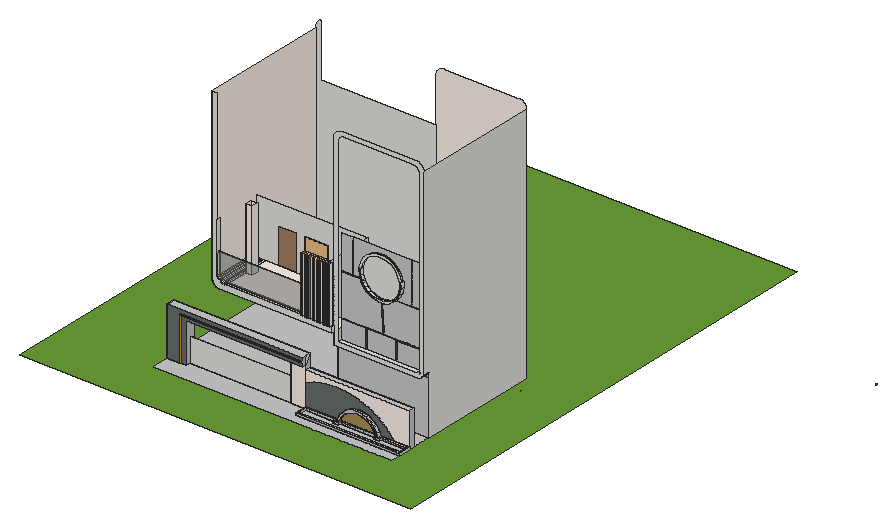
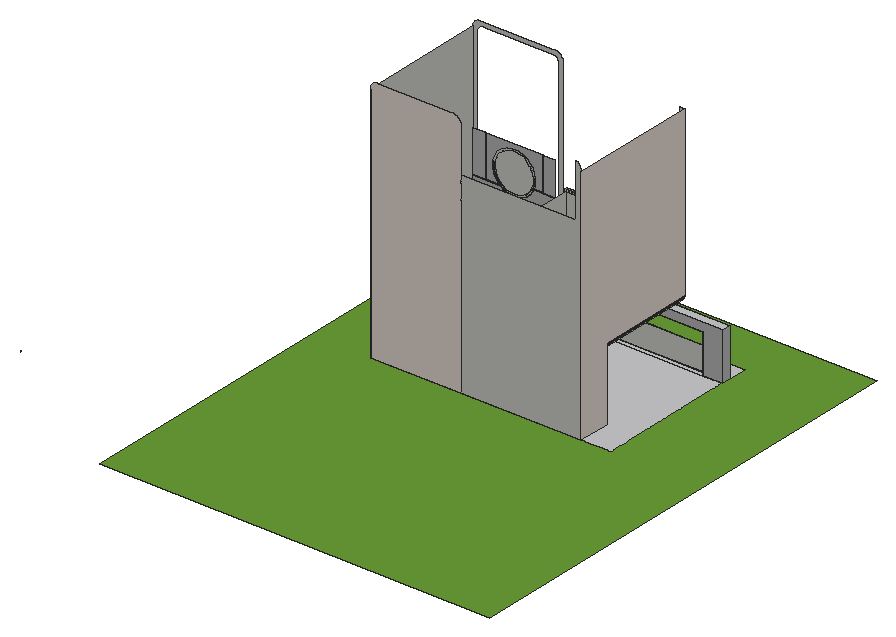
# SketchUp Ruby script. Lengths in inches.
U = 1.inch
M = Sketchup.active_model
def pt(a) = Geom::Point3d.new(a.map { |v| v * U })
def face(e, loops, mat)
  f = e.add_face(loops[0].map { |a| pt(a) })
  loops[1..].each { |l| e.add_face(l.map { |a| pt(a) }).erase! }
  f.material = f.back_material = mat if mat
  f
end
# faces: each face lists its corners as indices into pts; further lists are holes
def faces(e, pts, list, mat = nil) = list.each { |f| face(e, (f[0].is_a?(Array) ? f : [f]).map { |l| l.map { |i| pts[i] } }, mat) }
# xy, xz, yz: faces in a plane at the given z, y or x. An outline is a flat list of corners, or four numbers for a rectangle; further outlines are holes
def ring(l) = l.size == 4 ? [[l[0], l[1]], [l[2], l[1]], [l[2], l[3]], [l[0], l[3]]] : l.each_slice(2).to_a
def flat(e, list, mat, &to3) = list.each { |f| face(e, (f[0].is_a?(Array) ? f : [f]).map { |l| ring(l).map { |u, v| to3.(u, v) } }, mat) }
def xy(e, z, list, mat = nil) = flat(e, list, mat) { |x, y| [x, y, z] }
def xz(e, y, list, mat = nil) = flat(e, list, mat) { |x, z| [x, y, z] }
def yz(e, x, list, mat = nil) = flat(e, list, mat) { |y, z| [x, y, z] }
def lines(e, pts, list) = list.each { |a, b| e.add_line(pt(pts[a]), pt(pts[b])) }
# prism: a flat outline (further loops are holes) pulled along v
def prism(e, loops, v, mat = nil)
  f = face(e, loops, mat); d = Geom::Vector3d.new(v.map { |x| x * U })
  f.pushpull(f.normal.samedirection?(d) ? d.length : -d.length)
end
def box(e, o, s, mat = nil) = prism(e, [[o, [o[0] + s[0], o[1], o[2]], [o[0] + s[0], o[1] + s[1], o[2]], [o[0], o[1] + s[1], o[2]]]], [0, 0, s[2]], mat)
def at(x, y, z, deg = 0) = Geom::Transformation.translation(pt([x, y, z])) * Geom::Transformation.rotation(ORIGIN, Z_AXIS, deg.degrees)
def axes(o, x, y, z) = Geom::Transformation.new([*x, 0, *y, 0, *z, 0, *pt(o).to_a, 1])
def part(name) = M.definitions.add(name)
# library, detail: a bought-in or finely detailed component or shape, given as its bounding box
def library(name, o, s) = part(name).tap { |d| box(d.entities, o, s) }
def detail(e, o, s) = box(e.add_group.entities, o, s)
def put(e, d, t, mat = nil) = e.add_instance(d, t).tap { |i| i.material = mat if mat }
def group(e, t, mat = nil) = e.add_group.tap { |g| g.transformation = t; g.material = mat if mat }.entities
root = M.entities
M.materials.add("Polis06_194").color = [79, 50, 36]
M.materials.add("[0009_Linen]").color = [250, 240, 230]
M.materials.add("[0045_Goldenrod]").color = [218, 165, 32]
M.materials.add("[Asphalt New]").color = [67, 60, 62]
M.materials.add("[Brick Rough Tan]").color = [167, 141, 82]
M.materials.add("[Cladding Siding Tan]").color = [162, 126, 95]
M.materials.add("[Cladding Stucco White]").color = [200, 200, 200]
M.materials.add("[Grass Dark Green]").color = [106, 157, 55]
M.materials.add("[Polished Concrete New]").color = [200, 200, 203]
M.materials.add("[Slate]").color = [102, 110, 108]
M.materials.add("[Translucent Glass Gray]").color = [128, 128, 128]
M.materials["[Translucent Glass Gray]"].alpha = 0.5
M.materials.add("[Wood Bamboo]").color = [177, 105, 43]
M.materials.add("[Wood Floor]").color = [155, 105, 61]
c1 = part("群组\#3")
xy(c1.entities,0,[[0,0,4.72,1.18],[0,34.25,4.72,35.43]],"Polis06_194")
xy(c1.entities,85.26,[[0,1.18,4.72,34.25]],"Polis06_194")
xy(c1.entities,86.61,[[0,0,4.72,35.43]],"Polis06_194")
xz(c1.entities,0,[[0,0,4.72,86.61]],"Polis06_194")
xz(c1.entities,1.18,[[0,0,2.36,85.26],[2.36,0,4.72,85.26]],"Polis06_194")
xz(c1.entities,34.25,[[0,0,4.72,85.26]],"Polis06_194")
xz(c1.entities,35.43,[[0,0,4.72,86.61]],"Polis06_194")
yz(c1.entities,0,[[0,0,1.18,86.61],[34.25,0,35.43,86.61],[1.18,85.26,34.25,86.61]],"Polis06_194")
yz(c1.entities,2.36,[[1.18,0,34.25,0,34.25,85.21,1.18,85.26]],"Polis06_194")
yz(c1.entities,4.72,[[0,0,1.18,86.61],[34.25,0,35.43,86.61],[1.18,85.26,34.25,86.61]],"Polis06_194")
c2 = library("fronceur+aubin+blanc+(3) (1)",[-47.99,-0.29,1.66],[95.37,4.84,114.09])
xy(root,0,[[42322.46,33003.45,66023.61,33977.14],[48032.1875,37569.95,66023.61,37569.95,66023.61,61909.82,24094.5625,61909.82,24094.5625,55566.63,48032.1875,55566.63]])
xy(root,0,[[[0,18501.72,77772.5625,114656.97],[22107.09,33300.11,22107.09,33977.14,18219.3,33977.14,18219.3,61909.82,66023.61,61909.82,66023.61,33977.14,42322.46,33977.14,42322.46,33300.11],[18219.3,28436.95,18219.3,32203.32,20884.66,32203.32,20884.66,32008.2,20984.47,32008.2,20984.47,32203.32,22107.09,32203.32,22107.09,33090.23,42322.46,33090.23,42322.46,33003.45,45279.84,33003.45,45279.84,30424.78,66023.61,30424.78,66023.61,28436.95],[45621.59,30766.53,45621.59,32661.7,51304.59,32661.7,51304.59,32107.95,52490.63,32107.95,52490.63,32661.7,59444.32,32661.7,59444.32,32107.95,60630.36,32107.95,60630.36,32661.7,65681.86,32661.7,65681.86,30766.53],[59786.07,32449.7,60288.61,33003.45],[51646.34,32449.7,52148.88,33003.45]]],"[Grass Dark Green]")
xy(root,0,[[18219.3,28436.95,66023.61,28436.95,66023.61,30424.78,45279.84,30424.78,45279.84,33003.45,42322.46,33003.45,42322.46,33090.23,22107.09,33090.23,22107.09,32203.32,20984.47,32203.32,20984.47,32008.2,20884.66,32008.2,20884.66,32203.32,18219.3,32203.32],[45621.59,30766.53,65681.86,30766.53,65681.86,32661.7,60630.36,32661.7,60630.36,32107.95,59444.32,32107.95,59444.32,32661.7,52490.63,32661.7,52490.63,32107.95,51304.59,32107.95,51304.59,32661.7,45621.59,32661.7],[51646.34,32449.7,52148.88,33003.45],[59786.07,32449.7,60288.61,33003.45],[22107.09,33300.11,42322.46,33977.14],
  [18219.3,33977.14,66023.61,33977.14,66023.61,37569.95,48032.1875,37569.95,48032.1875,55566.63,24094.5625,55566.63,24094.5625,61909.82,18219.3,61909.82]],"[Polished Concrete New]")
xy(root,403.125,[[[45279.84,30424.78,66023.61,30424.78,66023.61,33003.45,60288.61,33003.45,60288.61,32449.7,59786.07,32449.7,59786.07,33003.45,52148.88,33003.45,52148.88,32449.7,51646.34,32449.7,51646.34,33003.45,45279.84,33003.45],[45621.59,30766.53,45621.59,32661.7,51304.59,32661.7,51304.59,32107.95,52490.63,32107.95,52490.63,32661.7,59444.32,32661.7,59444.32,32107.95,60630.36,32107.95,60630.36,32661.7,65681.86,32661.7,65681.86,30766.53]]],"[Polished Concrete New]")
xy(root,6973.375,[[45279.84,33003.45,66023.61,33977.14]],"[Polished Concrete New]")
xy(root,7836,[[22107.09,32203.32,22107.09,33977.14,42322.46,33977.14,42322.46,33003.45,45279.84,33003.45,45279.84,32203.32]],"[Polished Concrete New]")
xy(root,8670.53,[[20984.47,32008.2,45279.84,32203.32]],"[0045_Goldenrod]")
xy(root,8794.03,[[20884.66,32008.2,45279.84,32203.32]],"[0045_Goldenrod]")
xy(root,9505.0625,[[18219.3,32203.32,45279.84,33977.14]],"[Polished Concrete New]")
xy(root,10796.53,[[48032.1875,36436.82,64738.58,37569.95]])
xy(root,11608.96,[[48844.61,36436.82,64428.16,37569.95],[64428.16,36610.22,65187.54,36610.22,65211.19,37569.95,64428.16,37569.95],[65187.54,36610.22,65211.19,36610.22,65211.19,37569.95]])
xy(root,13116.08,[[25598.07,36109.95,25598.07,42633.68,26902.95,42633.68,26902.95,43938.55,25598.07,43938.55,25598.07,55566.63,48032.1875,55566.63,48032.1875,36109.95]],"[0009_Linen]")
xy(root,14269.25,[[26296.56,36109.95,26424.7,36851.76],[26890.7,36109.95,47071.94,36851.76]])
xy(root,14289.45,[[41914.25,35829.26,41914.25,36851.76,47071.94,36851.76,47071.94,35829.26,46862.23,35829.26,46862.23,36436.82,46652.53,36436.82,46652.53,35829.26,46362.66,35829.26,46362.66,36436.82,46078.9,36436.82,46078.9,35829.26,45797.6,35829.26,45797.6,36436.82,45537.5,36436.82,45537.5,35829.26,45185.32,35829.26,45185.32,36436.82,44725.28,36436.82,44725.28,35829.26,44363.15,35829.26,44363.15,36436.82,43975.34,36436.82,43975.34,35829.26,43484.85,35829.26,43484.85,36436.82,43218.625,36436.82,43218.625,35829.26,42781.34,35829.26,42781.34,36436.82,42429.61,36436.82,42429.61,35829.26]])
xy(root,14289.45,[[47071.94,35829.26,47214.9,36109.95],[47390.11,35829.26,47723.54,36109.95],[47214.9,36109.95,47390.11,36436.82],[47723.54,36109.95,48032.1875,36436.82]],"[0009_Linen]")
xz(root,30424.78,[[45279.84,0,66023.61,403.125]],"[Polished Concrete New]")
xz(root,30766.53,[[45621.59,0,65681.86,403.125]],"[Polished Concrete New]")
xz(root,32008.2,[[20884.66,0,20984.47,0,20984.47,8670.53,45279.84,8670.53,45279.84,8794.03,20884.66,8794.03]],"[0045_Goldenrod]")
xz(root,32107.95,[[51304.59,0,52490.63,403.125],[59444.32,0,60630.36,403.125]],"[Polished Concrete New]")
xz(root,32203.32,[[18219.3,0,20884.66,0,20884.66,8794.03,45279.84,8794.03,45279.84,9505.0625,18219.3,9505.0625],[20984.47,0,22107.09,0,22107.09,7836,45279.84,7836,45279.84,8670.53,20984.47,8670.53]],"[Slate]")
xz(root,32449.7,[[51646.34,0,51646.34,403.125,51791.59,403.125],[51646.34,0,52148.88,0,52148.88,403.125,51791.59,403.125],[52148.88,0,52444.68,820.93,52914.5,1556.25,53535.13,2169.63,54275.93,2630.78,55100.28,2916.9,55967.47,3013.875,56834.67,2916.9,57659.02,2630.78,58399.8125,2169.63,59020.45,1556.25,59490.27,820.93,59786.07,0,59786.07,403.125,60143.36,403.125,59917.14,1030.9375,59390.39,1855.36,58694.55,2543.07,57863.99,3060.09,56939.75,3380.89,55967.47,3489.61,54995.2,3380.89,54070.95,3060.09,53240.4,2543.07,52544.56,1855.36,52017.8,1030.9375,51791.59,403.125,52148.88,403.125],[59786.07,0,60288.61,0,60143.36,403.125,59786.07,403.125],[60288.61,0,60143.36,403.125,60288.61,403.125]],"[Polished Concrete New]")
xz(root,32661.7,[[45621.59,0,51304.59,403.125],[52490.63,0,59444.32,403.125],[60630.36,0,63156.11,403.125],[63156.11,0,65681.86,403.125]],"[Polished Concrete New]")
xz(root,33003.45,[[51475.98,-472.79,60458.96,-472.79,60288.61,0,51646.34,0],[51646.34,0,52148.88,0,52148.88,403.125,52294.13,403.125,52444.68,820.93,52914.5,1556.25,53535.13,2169.63,54275.93,2630.78,55100.28,2916.9,55967.47,3013.875,56834.67,2916.9,57659.02,2630.78,58399.8125,2169.63,59020.45,1556.25,59490.27,820.93,59640.8125,403.125,59786.07,403.125,59786.07,0,60288.61,0,59917.14,1030.9375,59390.39,1855.36,58694.55,2543.07,57863.99,3060.09,56939.75,3380.89,55967.47,3489.61,54995.2,3380.89,54070.95,3060.09,53240.4,2543.07,52544.56,1855.36,52017.8,1030.9375],[52148.88,0,52148.88,403.125,52294.13,403.125],[59786.07,0,59640.8125,403.125,59786.07,403.125]])
xz(root,33003.45,[[42322.46,0,45279.84,7836],[63156.11,0,63156.11,403.125,62835.32,403.125],[62835.32,403.125,66023.61,403.125,66023.61,6973.375,45279.84,6973.375,45279.84,4704.0625,46830.7,5330.75,48443.94,5772.76,50097.65,6024.07,51769.36,6081.28,53436.38,5943.6,55076.0625,5612.92,56666.14,5093.71,58185,4393.03,59612.04,3520.4,60927.85,2487.67,62114.58,1308.87]],"[0009_Linen]")
xz(root,33003.45,[[52148.88,0,59786.07,0,59640.8125,403.125,52294.13,403.125],[52294.13,403.125,59640.8125,403.125,59490.27,820.93,59020.45,1556.25,58399.8125,2169.63,57659.02,2630.78,56834.67,2916.9,55967.47,3013.875,55100.28,2916.9,54275.93,2630.78,53535.13,2169.63,52914.5,1556.25,52444.68,820.93]],"[Brick Rough Tan]")
xz(root,33003.45,[[45279.84,0,51646.34,403.125],[63156.11,0,66023.61,403.125]],"[Polished Concrete New]")
xz(root,33003.45,[[51646.34,0,52017.8,1030.9375,52544.56,1855.36,53240.4,2543.07,54070.95,3060.09,54995.2,3380.89,55967.47,3489.61,56939.75,3380.89,57863.99,3060.09,58694.55,2543.07,59390.39,1855.36,59917.14,1030.9375,60288.61,0,60288.61,403.125,62835.32,403.125,62114.58,1308.87,60927.85,2487.67,59612.04,3520.4,58185,4393.03,56666.14,5093.71,55076.0625,5612.92,53436.38,5943.6,51769.36,6081.28,50097.65,6024.07,48443.94,5772.76,46830.7,5330.75,45279.84,4704.0625,45279.84,403.125,51646.34,403.125],[60288.61,0,60288.61,403.125,62835.32,403.125,63156.11,0]],"[Slate]")
xz(root,33090.23,[[22107.09,0,42322.46,4773.73]])
xz(root,33977.14,[[18219.3,0,18219.3,9505.0625,45279.84,9505.0625,45279.84,6973.375,66023.61,6973.375,66023.61,0,42322.46,0,42322.46,7836,22107.09,7836,22107.09,0]],"[Polished Concrete New]")
xz(root,35829.26,[[41914.25,14289.45,42429.61,25308.0625],[42781.34,14289.45,43218.625,25308.0625],[43484.85,14289.45,43975.34,25308.0625],[44363.15,14289.45,44725.28,25308.0625],[45185.32,14289.45,45537.5,25308.0625],
  [45797.6,14289.45,46078.9,25308.0625],[46362.66,14289.45,46652.53,25308.0625],[46862.23,14289.45,47214.9,25308.0625],[47390.11,14289.45,47723.54,25308.0625]],"[Wood Bamboo]")
xz(root,36109.95,[[25598.07,13116.08,48032.1875,13116.08,48032.1875,14289.45,47071.94,14289.45,47071.94,14269.25,26890.7,14269.25,26692.32,14251.67,26493.28,14258.44,26424.7,14269.25,26296.56,14269.25,26296.56,14289.45,26105.09,14344.23,25921.74,14421.97,25749.24,14521.51,25590.18,14641.35,25446.9375,14779.71,25321.65,14934.52,25216.19,15103.46,25132.14,15284,25070.75,15473.46,25070.75,47832.33,24094.5625,47832.33,24094.5625,14373.51,24135.97,14201.18,24197.0625,14034.82,24277.01,13876.65,24374.74,13728.8,24488.94,13593.26,24618.07,13471.87,24760.38,13366.25,24913.98,13277.82,25076.78,13207.78,25246.6,13157.07,25421.14,13126.36]])
xz(root,36436.82,[[[48032.1875,10796.53,64738.58,10796.53,64870.39,10825.61,64999.77,10864.08,65126.06,10911.73,65248.59,10968.33,65366.75,11033.58,65479.92,11107.15,65587.52,11188.65,65688.98,11277.66,65783.8,11373.73,65871.47,11476.36,65951.54,11585.02,66023.61,11699.15,66023.61,47979.42,66011,48171.85,65973.375,48360.98,65911.39,48543.59,65826.09,48716.55,65718.96,48876.9,65591.81,49021.88,65446.82,49149.03,65286.47,49256.17,65113.52,49341.47,64930.91,49403.45,64741.77,49441.07,64549.34,49453.6875,49822.99,49453.6875,49589.24,49438.37,49359.49,49392.67,49137.68,49317.37,48927.59,49213.77,48732.82,49083.625,48556.7,48929.17,48402.25,48753.06,48272.11,48558.29,48168.5,48348.2,48093.21,48126.38,48047.51,47896.63,48032.1875,47662.89],[48844.61,11608.96,48844.61,47320.58,48850.91,47456.76,48869.76,47591.78,48901,47724.48,48944.36,47853.73,48999.48,47978.42,49065.87,48097.49,49142.97,48209.92,49230.13,48314.75,49326.6,48411.08,49431.55,48498.1,49544.09,48575.04,49663.25,48641.27,63903.99,48641.27,64070.97,48630.32,64235.09,48597.68,64393.55,48543.89,64543.625,48469.875,64682.76,48376.91,64808.57,48266.58,64918.91,48140.76,65011.875,48001.63,65085.89,47851.55,65139.68,47693.09,65172.32,47528.97,65183.27,47361.99,65183.27,12216.36,65148.81,12114.85,65101.4,12018.71,65041.84,11929.58,64971.16,11848.98,64890.57,11778.3,64801.43,11718.75,64705.29,11671.34,64603.78,11636.88,64498.65,11615.97,64391.68,11608.96]]])
xz(root,36436.82,[[47723.54,14289.45,48032.1875,25308.0625]],"[0009_Linen]")
xz(root,36436.82,[[42429.61,14289.45,42781.34,25308.0625],[43218.625,14289.45,43484.85,25308.0625],[43975.34,14289.45,44363.15,25308.0625],[44725.28,14289.45,45185.32,25308.0625],[45537.5,14289.45,45797.6,25308.0625],
  [46078.9,14289.45,46362.66,25308.0625],[46652.53,14289.45,46862.23,25308.0625],[47214.9,14289.45,47390.11,25308.0625]],"[Translucent Glass Gray]")
xz(root,36480.85,[[25085.58,14266.82,25078.51,19525.13,41907.18,19547.75,41914.25,14289.45,26890.7,14269.25]],"[Translucent Glass Gray]")
xz(root,36851.76,[[26692.32,14251.67,26890.7,14269.25,26424.7,14269.25,26493.28,14258.44],[26296.56,14269.25,26424.7,14269.25,26296.56,14289.45],[26424.7,14269.25,47071.94,14269.25,47071.94,14289.45,26296.56,14289.45],[41914.25,14289.45,47071.94,25308.0625]])
xz(root,37043.95,[[[56489.97,21300.85,57592.81,21343.51,58647.03,21670.15,59580.79,22258.51,60330.45,23068.5,60844.93,24044.91,61089.16,25121.21,61046.5,26224.05,60719.86,27278.27,60131.5,28212.03,59321.51,28961.69,58345.1,29476.17,57268.8,29720.41,56165.96,29677.75,55111.74,29351.11,54177.98,28762.75,53428.32,27952.76,52913.84,26976.35,52669.6,25900.04,52712.26,24797.2,53038.9,23742.98,53627.26,22809.22,54437.25,22059.5625,55413.66,21545.08],[56519.82,21623.61,55526.04,21849.12,54624.48,22324.15,53876.6,23016.34,53333.34,23878.51,53031.75,24851.9,52992.36,25870.1875,53217.87,26863.97,53692.9,27765.53,54385.09,28513.41,55247.26,29056.67,56220.66,29358.26,57238.94,29397.65,58232.73,29172.14,59134.28,28697.11,59882.17,28004.92,60425.42,27142.75,60727.02,26169.35,60766.4,25151.07,60540.89,24157.29,60065.86,23255.73,59373.67,22507.84,58511.5,21964.59,57538.11,21662.99]]])
xz(root,37569.95,[[[56489.97,21300.85,56815.88,21313.46,57041.39,21322.18,57592.81,21343.51,58647.03,21670.15,59580.79,22258.51,59580.79,22374.64,59688.26,22374.64,60330.45,23068.5,60844.93,24044.91,61089.16,25121.21,61046.5,26224.05,60719.86,27278.27,60131.5,28212.03,59321.51,28961.69,58345.1,29476.17,57268.8,29720.41,56165.96,29677.75,55111.74,29351.11,54177.98,28762.75,53428.32,27952.76,52913.84,26976.35,52669.6,25900.04,52712.26,24797.2,52976.39,23944.74,53038.9,23944.74,53038.9,23742.98,53627.26,22809.22,54437.25,22059.5625,55413.66,21545.08],[56519.82,21623.61,55526.04,21849.12,54624.48,22324.15,53876.6,23016.34,53333.34,23878.51,53031.75,24851.9,52992.36,25870.1875,53217.87,26863.97,53692.9,27765.53,54385.09,28513.41,55247.26,29056.67,56220.66,29358.26,57238.94,29397.65,58232.73,29172.14,59134.28,28697.11,59882.17,28004.92,60425.42,27142.75,60727.02,26169.35,60766.4,25151.07,60540.89,24157.29,60065.86,23255.73,59373.67,22507.84,58511.5,21964.59,57538.11,21662.99]],[56519.82,21623.61,57538.11,21662.99,58511.5,21964.59,59373.67,22507.84,60065.86,23255.73,60540.89,24157.29,60766.4,25151.07,60727.02,26169.35,60425.42,27142.75,59882.17,28004.92,59134.28,28697.11,58232.73,29172.14,57238.94,29397.65,56220.66,29358.26,55247.26,29056.67,54385.09,28513.41,53692.9,27765.53,53217.87,26863.97,52992.36,25870.1875,53031.75,24851.9,53333.34,23878.51,53876.6,23016.34,54624.48,22324.15,55526.04,21849.12],[59580.79,22258.51,59688.26,22374.64,59580.79,22374.64],[53038.9,23742.98,53038.9,23944.74,52976.39,23944.74]])
xz(root,37569.95,[[53528,11608.96,53697.9,15066.51],[59580.79,11841.43,59759.1,15272.35],[48844.61,15272.35,59580.79,15483.18],[59580.79,15272.35,59759.1,15483.18],[59759.1,15272.35,65211.19,15483.18],
  [57041.39,15483.18,57266.89,15491.91,57041.39,21322.18,56815.88,21313.46],[59580.79,22258.51,65211.19,22258.51,65211.19,22374.64,59688.26,22374.64],[62553.91,22374.64,62791.13,30695.54],[48844.61,23742.98,53038.9,23742.98,52976.39,23944.74,48844.61,23944.74],[50910.5,23944.74,51149.6,30695.54]],"[Asphalt New]")
xz(root,37569.95,[[48032.1875,0,66023.61,10796.53],[64738.58,10796.53,66023.61,10796.53,66023.61,11699.15,65951.54,11585.02,65871.47,11476.36,65783.8,11373.73,65688.98,11277.66,65587.52,11188.65,65479.92,11107.15,65366.75,11033.58,65248.59,10968.33,65126.06,10911.73,64999.77,10864.08,64870.39,10825.61]],"[Cladding Stucco White]")
xz(root,37569.95,[[48844.61,11608.96,53528,11608.96,53528,15066.51,53697.9,15066.51,53697.9,11608.96,65211.19,11608.96,65211.19,15272.35,59759.1,15272.35,59759.1,11841.43,59580.79,11841.43,59580.79,15272.35,48844.61,15272.35],[48844.61,15483.18,57041.39,15483.18,56815.88,21313.46,56489.97,21300.85,55413.66,21545.08,54437.25,22059.5625,53627.26,22809.22,53038.9,23742.98,48844.61,23742.98],[57041.39,15483.18,65211.19,15483.18,65211.19,22258.51,59580.79,22258.51,58647.03,21670.15,57592.81,21343.51,57041.39,21322.18,57266.89,15491.91],[59688.26,22374.64,62553.91,22374.64,62553.91,30695.54,51149.6,30695.54,51149.6,23944.74,52976.39,23944.74,52712.26,24797.2,52669.6,25900.04,52913.84,26976.35,53428.32,27952.76,54177.98,28762.75,55111.74,29351.11,56165.96,29677.75,57268.8,29720.41,58345.1,29476.17,59321.51,28961.69,60131.5,28212.03,60719.86,27278.27,61046.5,26224.05,61089.16,25121.21,60844.93,24044.91,60330.45,23068.5],[62791.13,22374.64,65211.19,30695.54],
  [48844.61,23944.74,50910.5,30695.54]],"[Polished Concrete New]")
xz(root,42633.68,[[25598.07,13116.08,26902.95,25456.33]],"[0009_Linen]")
xz(root,43938.55,[[25598.07,13116.08,26902.95,25456.33]],"[0009_Linen]")
xz(root,46071.33,[[25070.75,14269.25,29233.36,14269.25,29233.36,21342.75,33009.3,21342.75,33009.3,14269.25,34611.99,14269.25,34611.99,21330.28,38975.95,21330.28,38975.95,14269.25,47071.94,14269.25,47071.94,25308.0625,25070.75,25308.0625],[[29233.36,14269.25,33009.3,21342.75],[29360.15,14396.05,32882.5,21215.95]]])
xz(root,46071.33,[[[34611.99,14269.25,38975.95,21330.28],[34795.89,14453.15,38792.05,21146.38]],[36793.97,14453.15,37002.21,18203.375],[34795.89,18203.375,36793.97,18489.67],[36793.97,18203.375,37002.21,18489.67],[37002.21,18203.375,38792.05,18489.67],
  [36793.97,18489.67,37002.21,21146.38]],"[Asphalt New]")
xz(root,46071.33,[[29360.15,14396.05,32882.5,21215.95]],"[Cladding Siding Tan]")
xz(root,46071.33,[[34795.89,14453.15,36793.97,18203.375],[37002.21,14453.15,38792.05,18203.375],[34795.89,18489.67,36793.97,21146.38],[37002.21,18489.67,38792.05,21146.38]],"[Translucent Glass Gray]")
xz(root,55566.63,[[[24094.5625,0,30467.68,0,30467.68,10401.79,36063.375,10401.79,36063.375,0,48032.1875,0,48032.1875,13116.08,24094.5625,13116.08],[40784.11,3703.3125,44855.24,10290.53]],[24094.5625,13116.08,25598.07,13116.08,25421.14,13126.36,25246.6,13157.07,25076.78,13207.78,24913.98,13277.82,24760.38,13366.25,24618.07,13471.87,24488.94,13593.26,24374.74,13728.8,24277.01,13876.65,24197.0625,14034.82,24135.97,14201.18,24094.5625,14373.51]])
xz(root,55566.63,[[[40784.11,3703.3125,44855.24,10290.53],[41037.36,3956.57,44601.98,10037.28]],[41037.36,6741.3125,44601.98,6996.92]],"[Asphalt New]")
xz(root,55566.63,[[41037.36,3956.57,44601.98,6741.3125],[41037.36,6996.92,44601.98,10037.28]],"[Translucent Glass Gray]")
xz(root,55566.63,[[30634.6,166.92,35896.46,10234.875]],"[Wood Bamboo]")
xz(root,55566.63,[[[30467.68,0,36063.375,10401.79],[30634.6,166.92,35896.46,10234.875]]],"[Wood Floor]")
xz(root,61909.82,[[24094.5625,0,24094.5625,47832.33,24113.14,47986.375,24141.44,48138.93,24179.36,48289.39,24226.75,48437.14,24283.4,48581.59,24349.11,48722.15,24423.59,48858.27,24506.56,48989.39,24597.67,49114.98,24696.56,49234.55,24802.83,49347.6,24916.0625,49453.6875,25070.75,49453.6875,25070.75,38958,48032.1875,38958,48032.1875,0]])
xz(root,61909.82,[[48032.1875,0,48032.1875,47662.89,48047.51,47896.63,48093.21,48126.38,48168.5,48348.2,48272.11,48558.29,48402.25,48753.06,48556.7,48929.17,48732.82,49083.625,48927.59,49213.77,49137.68,49317.37,49359.49,49392.67,49589.24,49438.37,49822.99,49453.6875,64549.34,49453.6875,64741.77,49441.07,64930.91,49403.45,65113.52,49341.47,65286.47,49256.17,65446.82,49149.03,65591.81,49021.88,65718.96,48876.9,65826.09,48716.55,65911.39,48543.59,65973.375,48360.98,66011,48171.85,66023.61,47979.42,66023.61,0]],"[0009_Linen]")
yz(root,18219.3,[[32203.32,0,33977.14,9505.0625]],"[Polished Concrete New]")
yz(root,20884.66,[[32008.2,0,32203.32,8794.03]],"[0045_Goldenrod]")
yz(root,20984.47,[[32008.2,0,32203.32,8670.53]],"[0045_Goldenrod]")
yz(root,22107.09,[[32203.32,0,33090.23,0,33090.23,5590.25,33300.11,5590.25,33300.11,0,33977.14,0,33977.14,7836,32203.32,7836]],"[Polished Concrete New]")
yz(root,24094.5625,[[55566.63,0,55566.63,14373.51,36109.95,14373.51,36109.95,47832.33,61909.82,47832.33,61909.82,0]],"[0009_Linen]")
yz(root,25070.75,[[36109.95,15473.46,36851.76,25308.0625]])
yz(root,25598.07,[[42633.68,13116.08,43938.55,25456.33]],"[0009_Linen]")
yz(root,26296.56,[[36109.95,14269.25,36851.76,14289.45]])
yz(root,26902.95,[[42633.68,13116.08,43938.55,25456.33]],"[0009_Linen]")
yz(root,41914.25,[[35829.26,14289.45,36851.76,25308.0625]],"[Wood Bamboo]")
yz(root,42322.46,[[33003.45,0,33003.45,7836,33977.14,7836,33977.14,0,33300.11,0,33300.11,5590.25,33090.23,5590.25,33090.23,0],[33090.23,0,33300.11,5590.25]],"[Polished Concrete New]")
yz(root,42429.61,[[35829.26,14289.45,36436.82,25308.0625]],"[0009_Linen]")
yz(root,42781.34,[[35829.26,14289.45,36436.82,25308.0625]],"[Wood Bamboo]")
yz(root,43218.625,[[35829.26,14289.45,36436.82,25308.0625]],"[0009_Linen]")
yz(root,43484.85,[[35829.26,14289.45,36436.82,25308.0625]],"[Wood Bamboo]")
yz(root,43975.34,[[35829.26,14289.45,36436.82,25308.0625]],"[0009_Linen]")
yz(root,44363.15,[[35829.26,14289.45,36436.82,25308.0625]],"[Wood Bamboo]")
yz(root,44725.28,[[35829.26,14289.45,36436.82,25308.0625]],"[0009_Linen]")
yz(root,45185.32,[[35829.26,14289.45,36436.82,25308.0625]],"[Wood Bamboo]")
yz(root,45279.84,[[33003.45,7836,33977.14,9505.0625,33003.45,9505.0625]])
yz(root,45279.84,[[30424.78,0,33003.45,403.125],[33003.45,6973.375,33977.14,6973.375,33977.14,9505.0625,33003.45,7836],[32203.32,7836,33003.45,7836,33003.45,9505.0625,32203.32,9505.0625,32203.32,8794.03,32008.2,8794.03,32008.2,8670.53,32203.32,8670.53]],"[Polished Concrete New]")
yz(root,45537.5,[[35829.26,14289.45,36436.82,25308.0625]],"[0009_Linen]")
yz(root,45621.59,[[30766.53,0,32661.7,403.125]],"[Polished Concrete New]")
yz(root,45797.6,[[35829.26,14289.45,36436.82,25308.0625]],"[Wood Bamboo]")
yz(root,46078.9,[[35829.26,14289.45,36436.82,25308.0625]],"[0009_Linen]")
yz(root,46362.66,[[35829.26,14289.45,36436.82,25308.0625]],"[Wood Bamboo]")
yz(root,46652.53,[[35829.26,14289.45,36436.82,25308.0625]],"[0009_Linen]")
yz(root,46862.23,[[35829.26,14289.45,36436.82,25308.0625]],"[Wood Bamboo]")
yz(root,47071.94,[[36109.95,14269.25,36851.76,14289.45],[36851.76,14269.25,46071.33,25308.0625]])
yz(root,47214.9,[[35829.26,14289.45,36436.82,25308.0625]],"[0009_Linen]")
yz(root,47390.11,[[35829.26,14289.45,36436.82,25308.0625]],"[Wood Bamboo]")
yz(root,47723.54,[[35829.26,14289.45,36436.82,25308.0625]],"[0009_Linen]")
yz(root,48032.1875,[[37569.95,0,37569.95,10796.53,36436.82,10796.53,36436.82,13116.08,55566.63,13116.08,55566.63,0],[36109.95,13116.08,36436.82,14289.45]])
yz(root,51304.59,[[32107.95,0,32661.7,403.125]],"[Polished Concrete New]")
yz(root,51646.34,[[32449.7,0,33003.45,403.125]],"[Polished Concrete New]")
yz(root,52148.88,[[32449.7,0,33003.45,403.125]],"[Polished Concrete New]")
yz(root,52490.63,[[32107.95,0,32661.7,403.125]],"[Polished Concrete New]")
yz(root,59444.32,[[32107.95,0,32661.7,403.125]],"[Polished Concrete New]")
yz(root,59786.07,[[32449.7,0,33003.45,403.125]],"[Polished Concrete New]")
yz(root,60288.61,[[32449.7,0,33003.45,403.125]],"[Polished Concrete New]")
yz(root,60630.36,[[32107.95,0,32661.7,403.125]],"[Polished Concrete New]")
yz(root,65681.86,[[30766.53,0,32661.7,403.125]],"[Polished Concrete New]")
yz(root,66023.61,[[37569.95,0,61909.82,0,61909.82,47979.42,36436.82,47979.42,36436.82,11699.15,37569.95,11699.15]])
yz(root,66023.61,[[30424.78,0,33003.45,403.125],[33003.45,0,33977.14,6973.375]],"[Polished Concrete New]")
p = [[52017.8,33003.45,1030.9375],[51646.34,33003.45,0],[51646.34,32449.7,0],[51791.59,32449.7,403.125],[52017.8,32449.7,1030.9375],[52148.88,33003.45,0],
  [52294.13,33003.45,403.125],[52444.68,33003.45,820.93],[52444.68,32449.7,820.93],[52148.88,32449.7,0],[59490.27,33003.45,820.93],[59640.8125,33003.45,403.125],
  [59786.07,33003.45,0],[59786.07,32449.7,0],[59490.27,32449.7,820.93],[60288.61,33003.45,0],[59917.14,33003.45,1030.9375],[59917.14,32449.7,1030.9375],
  [60143.36,32449.7,403.125],[60288.61,32449.7,0],[52914.5,33003.45,1556.25],[52914.5,32449.7,1556.25],[59020.45,33003.45,1556.25],[59020.45,32449.7,1556.25],
  [52544.56,33003.45,1855.36],[52544.56,32449.7,1855.36],[59390.39,33003.45,1855.36],[59390.39,32449.7,1855.36],[53535.13,33003.45,2169.63],[53535.13,32449.7,2169.63],
  [58399.8125,33003.45,2169.63],[58399.8125,32449.7,2169.63],[53240.4,33003.45,2543.07],[53240.4,32449.7,2543.07],[58694.55,33003.45,2543.07],[58694.55,32449.7,2543.07],
  [54275.93,33003.45,2630.78],[54275.93,32449.7,2630.78],[57659.02,33003.45,2630.78],[57659.02,32449.7,2630.78],[54070.95,33003.45,3060.09],[54070.95,32449.7,3060.09],
  [57863.99,33003.45,3060.09],[57863.99,32449.7,3060.09],[55100.28,33003.45,2916.9],[55100.28,32449.7,2916.9],[56834.67,33003.45,2916.9],[56834.67,32449.7,2916.9],
  [55967.47,33003.45,3013.875],[55967.47,32449.7,3013.875],[54995.2,33003.45,3380.89],[54995.2,32449.7,3380.89],[56939.75,33003.45,3380.89],[56939.75,32449.7,3380.89],
  [55967.47,33003.45,3489.61],[55967.47,32449.7,3489.61],[64870.39,36436.82,10825.61],[64738.58,36436.82,10796.53],[64738.58,37569.95,10796.53],[64870.39,37569.95,10825.61],
  [64999.77,36436.82,10864.08],[64999.77,37569.95,10864.08],[65126.06,36436.82,10911.73],[65126.06,37569.95,10911.73],[65248.59,36436.82,10968.33],[65248.59,37569.95,10968.33],
  [65366.75,36436.82,11033.58],[65366.75,37569.95,11033.58],[65479.92,36436.82,11107.15],[65479.92,37569.95,11107.15],[65587.52,36436.82,11188.65],[65587.52,37569.95,11188.65],
  [65688.98,36436.82,11277.66],[65688.98,37569.95,11277.66],[65783.8,36436.82,11373.73],[65783.8,37569.95,11373.73],[65871.47,36436.82,11476.36],[65871.47,37569.95,11476.36],
  [65951.54,36436.82,11585.02],[65951.54,37569.95,11585.02],[66023.61,36436.82,11699.15],[66023.61,37569.95,11699.15],[65211.19,37569.95,12216.36],[65211.19,37569.95,11608.96],
  [65187.54,36610.22,11608.96],[65186.98,36587.44,11608.96],[65186.98,36587.44,12216.36],[25598.07,42633.68,13116.08],[25598.07,36109.95,13116.08],[25421.14,36109.95,13126.36],
  [25421.14,55566.63,13126.36],[25598.07,55566.63,13116.08],[25598.07,43938.55,13116.08],[25246.6,36109.95,13157.07],[25246.6,55566.63,13157.07],[25076.78,36109.95,13207.78],
  [25076.78,55566.63,13207.78],[24913.98,36109.95,13277.82],[24913.98,55566.63,13277.82],[24760.38,36109.95,13366.25],[24760.38,55566.63,13366.25],[24618.07,36109.95,13471.87],
  [24618.07,55566.63,13471.87],[24488.94,36109.95,13593.26],[24488.94,55566.63,13593.26],[24374.74,36109.95,13728.8],[24374.74,55566.63,13728.8],[24277.01,36109.95,13876.65],
  [24277.01,55566.63,13876.65],[24197.0625,36109.95,14034.82],[24197.0625,55566.63,14034.82],[24135.97,36109.95,14201.18],[24135.97,55566.63,14201.18],[24094.5625,36109.95,14373.51],
  [24094.5625,55566.63,14373.51],[26692.32,36851.76,14251.67],[26493.28,36851.76,14258.44],[26493.28,36109.95,14258.44],[26692.32,36109.95,14251.67],[26890.7,36851.76,14269.25],
  [26890.7,36109.95,14269.25],[26890.7,36340.51,14269.25],[26890.7,36480.85,14269.25],[26424.7,36851.76,14269.25],[26424.7,36109.95,14269.25],[25085.58,36480.85,14266.82],
  [25085.58,36340.51,14266.82],[25078.51,36340.51,19525.13],[25078.51,36480.85,19525.13],[41914.25,36340.51,14289.45],[41914.25,36480.85,14289.45],[26296.56,36851.76,14289.45],
  [26105.09,36851.76,14344.23],[26105.09,36109.95,14344.23],[26296.56,36109.95,14289.45],[41907.18,36480.85,19547.75],[41907.18,36340.51,19547.75],[25921.74,36851.76,14421.97],
  [25921.74,36109.95,14421.97],[25749.24,36851.76,14521.51],[25749.24,36109.95,14521.51],[25590.18,36851.76,14641.35],[25590.18,36109.95,14641.35],[25446.9375,36851.76,14779.71],
  [25446.9375,36109.95,14779.71],[25321.65,36851.76,14934.52],[25321.65,36109.95,14934.52],[25216.19,36851.76,15103.46],[25216.19,36109.95,15103.46],[25132.14,36851.76,15284],
  [25132.14,36109.95,15284],[25070.75,36851.76,15473.46],[25070.75,36109.95,15473.46],[55413.66,37569.95,21545.08],[56489.97,37569.95,21300.85],[56489.97,37043.95,21300.85],
  [55413.66,37043.95,21545.08],[57041.39,37569.95,21322.18],[57592.81,37569.95,21343.51],[57592.81,37043.95,21343.51],[56815.88,37569.95,21313.46],[58647.03,37569.95,21670.15],
  [58647.03,37043.95,21670.15],[54437.25,37569.95,22059.5625],[54437.25,37043.95,22059.5625],[56519.82,37569.95,21623.61],[55526.04,37569.95,21849.12],[55526.04,37043.95,21849.12],
  [56519.82,37043.95,21623.61],[57538.11,37569.95,21662.99],[57538.11,37043.95,21662.99],[58511.5,37569.95,21964.59],[58511.5,37043.95,21964.59],[59580.79,37569.95,22258.51],
  [59580.79,37043.95,22258.51],[54624.48,37569.95,22324.15],[54624.48,37043.95,22324.15],[59373.67,37569.95,22507.84],[59373.67,37043.95,22507.84],[53627.26,37569.95,22809.22],
  [53627.26,37043.95,22809.22],[59688.26,37569.95,22374.64],[60330.45,37569.95,23068.5],[60330.45,37043.95,23068.5],[53876.6,37569.95,23016.34],[53876.6,37043.95,23016.34],
  [60065.86,37569.95,23255.73],[60065.86,37043.95,23255.73],[53038.9,37569.95,23742.98],[53038.9,37043.95,23742.98],[53333.34,37569.95,23878.51],[53333.34,37043.95,23878.51],
  [60844.93,37569.95,24044.91],[60844.93,37043.95,24044.91],[60540.89,37569.95,24157.29],[60540.89,37043.95,24157.29],[52976.39,37569.95,23944.74],[52712.26,37043.95,24797.2],
  [52712.26,37569.95,24797.2],[53031.75,37569.95,24851.9],[53031.75,37043.95,24851.9],[61089.16,37569.95,25121.21],[61089.16,37043.95,25121.21],[60766.4,37569.95,25151.07],
  [60766.4,37043.95,25151.07],[52669.6,37569.95,25900.04],[52669.6,37043.95,25900.04],[52992.36,37569.95,25870.1875],[52992.36,37043.95,25870.1875],[61046.5,37569.95,26224.05],
  [61046.5,37043.95,26224.05],[60727.02,37569.95,26169.35],[60727.02,37043.95,26169.35],[25070.75,46071.33,14269.25],[25070.75,36851.76,14269.25],[65183.27,36436.82,12216.36],
  [65204.18,36436.82,12321.5],[65211.19,36436.82,12428.47],[65211.19,36610.22,11608.96],[65211.19,36436.82,11608.96],[22107.09,33090.23,4773.73],[42322.46,33003.45,4905.17]]
faces(root,p,[[0,1,2,3,4],[5,6,7,8,9],[10,11,12,13,14],[15,16,17,18,19],[7,20,21,8],[22,10,14,23],[24,0,4,25],[16,26,27,17],
  [20,28,29,21],[30,22,23,31],[32,24,25,33],[26,34,35,27],[28,36,37,29],[38,30,31,39],[40,32,33,41],[34,42,43,35],
  [36,44,45,37],[46,38,39,47],[44,48,49,45],[48,46,47,49],[50,40,41,51],[42,52,53,43],[54,50,51,55],[52,54,55,53]],"[Polished Concrete New]")
faces(root,p,[[56,57,58,59],[60,56,59,61],[62,60,61,63],[64,62,63,65],[66,64,65,67],[68,66,67,69],[70,68,69,71],[72,70,71,73],
  [74,72,73,75],[76,74,75,77],[78,76,77,79],[80,78,79,81],[82,83,84,85,86],[115,116,117,118],[119,115,118,120,121,122],[116,123,124,117],
  [125,126,127,128],[122,121,126,125],[129,121,122,130],[131,132,133,134],[129,130,135,136],[132,137,138,133],[137,139,140,138],[139,141,142,140],
  [141,143,144,142],[143,145,146,144],[145,147,148,146],[147,149,150,148],[149,151,152,150],[127,136,135,128],[153,154,155,156],[157,158,159,155,154,160],
  [158,161,162,159],[163,153,156,164],[165,166,167,168],[169,165,168,170],[171,169,170,172],[161,173,174,162],[166,175,176,167],[177,171,172,178],
  [179,163,164,180],[181,182,183,174,173],[175,184,185,176],[186,177,178,187],[188,179,180,189],[184,190,191,185],[182,192,193,183],[194,186,187,195],
  [196,188,189,197,198],[190,199,200,191],[192,201,202,193],[203,194,195,204],[205,198,197,206],[199,207,208,200],[201,209,210,202],[211,203,204,212]])
faces(root,p,[[87,88,89,90,91,92],[90,89,93,94],[94,93,95,96],[96,95,97,98],[98,97,99,100],[100,99,101,102],[102,101,103,104],[104,103,105,106],
  [106,105,107,108],[108,107,109,110],[110,109,111,112],[112,111,113,114]],"[0009_Linen]")
lines(root,p,[[213,214],[215,216],[216,217],[215,86],[218,219],[220,221]])
put(root,c1,at(67887.55,58297.69,0))
put(root,c2,at(109763.28,94352.92,0))
put(root,c2,axes([37022.1,46684.01,14004.78],[47.8192,0,0],[0,-151.6372,0],[0,0,62.92]))
